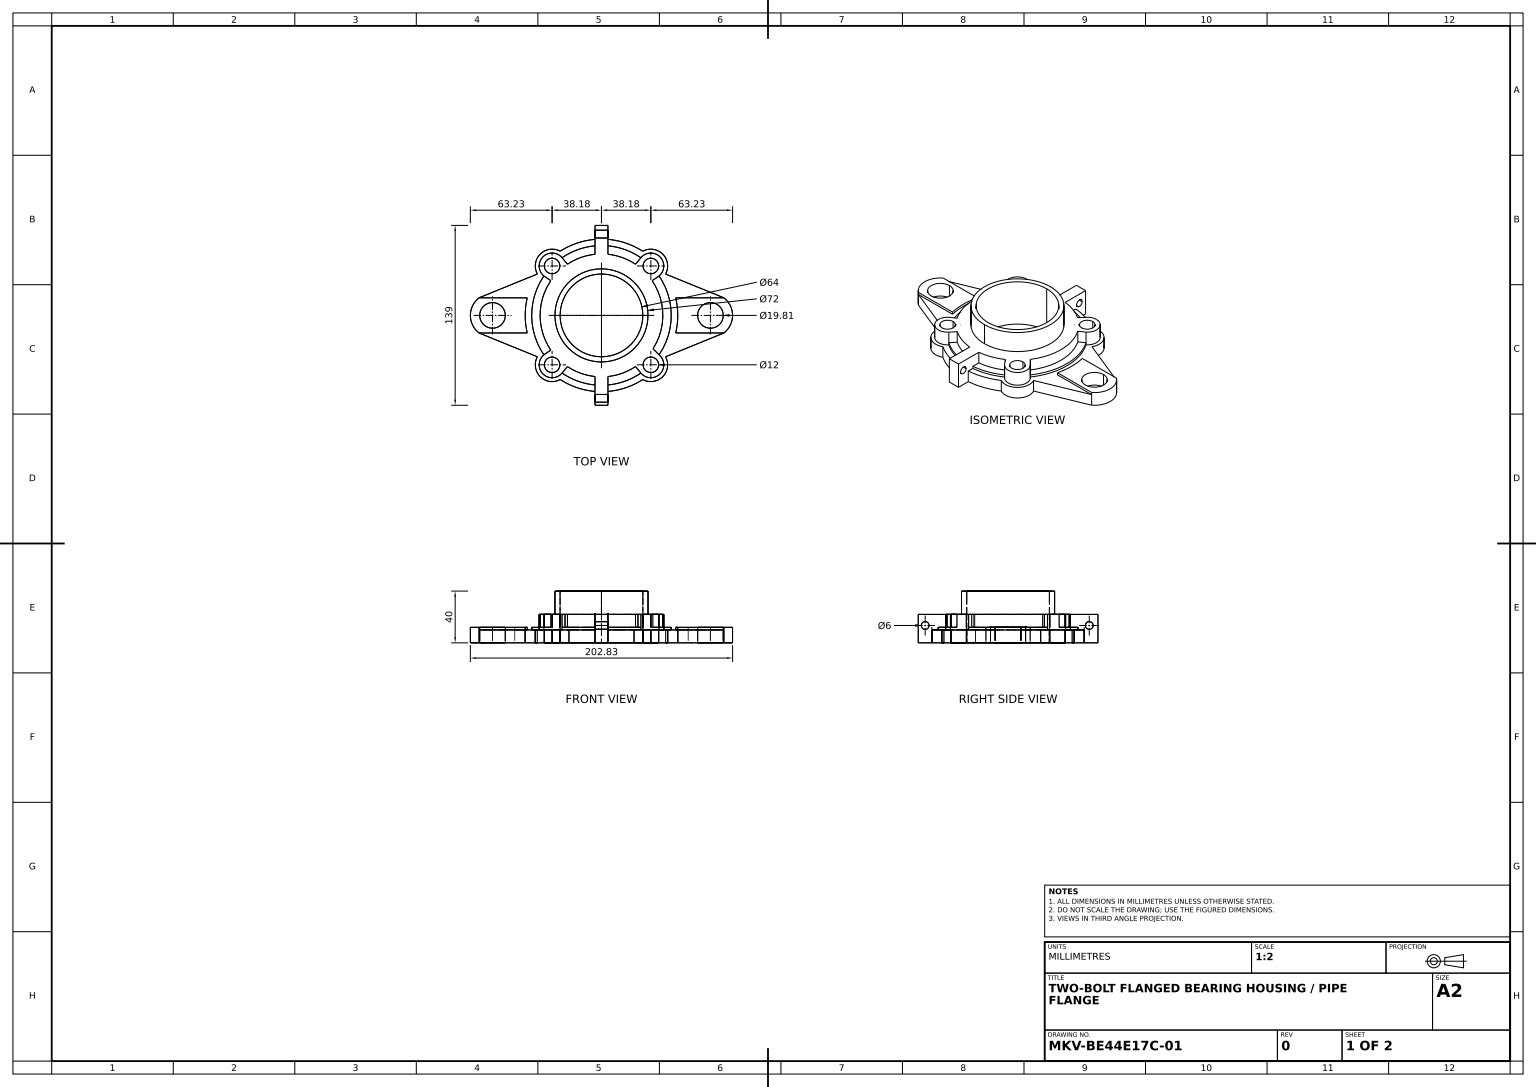
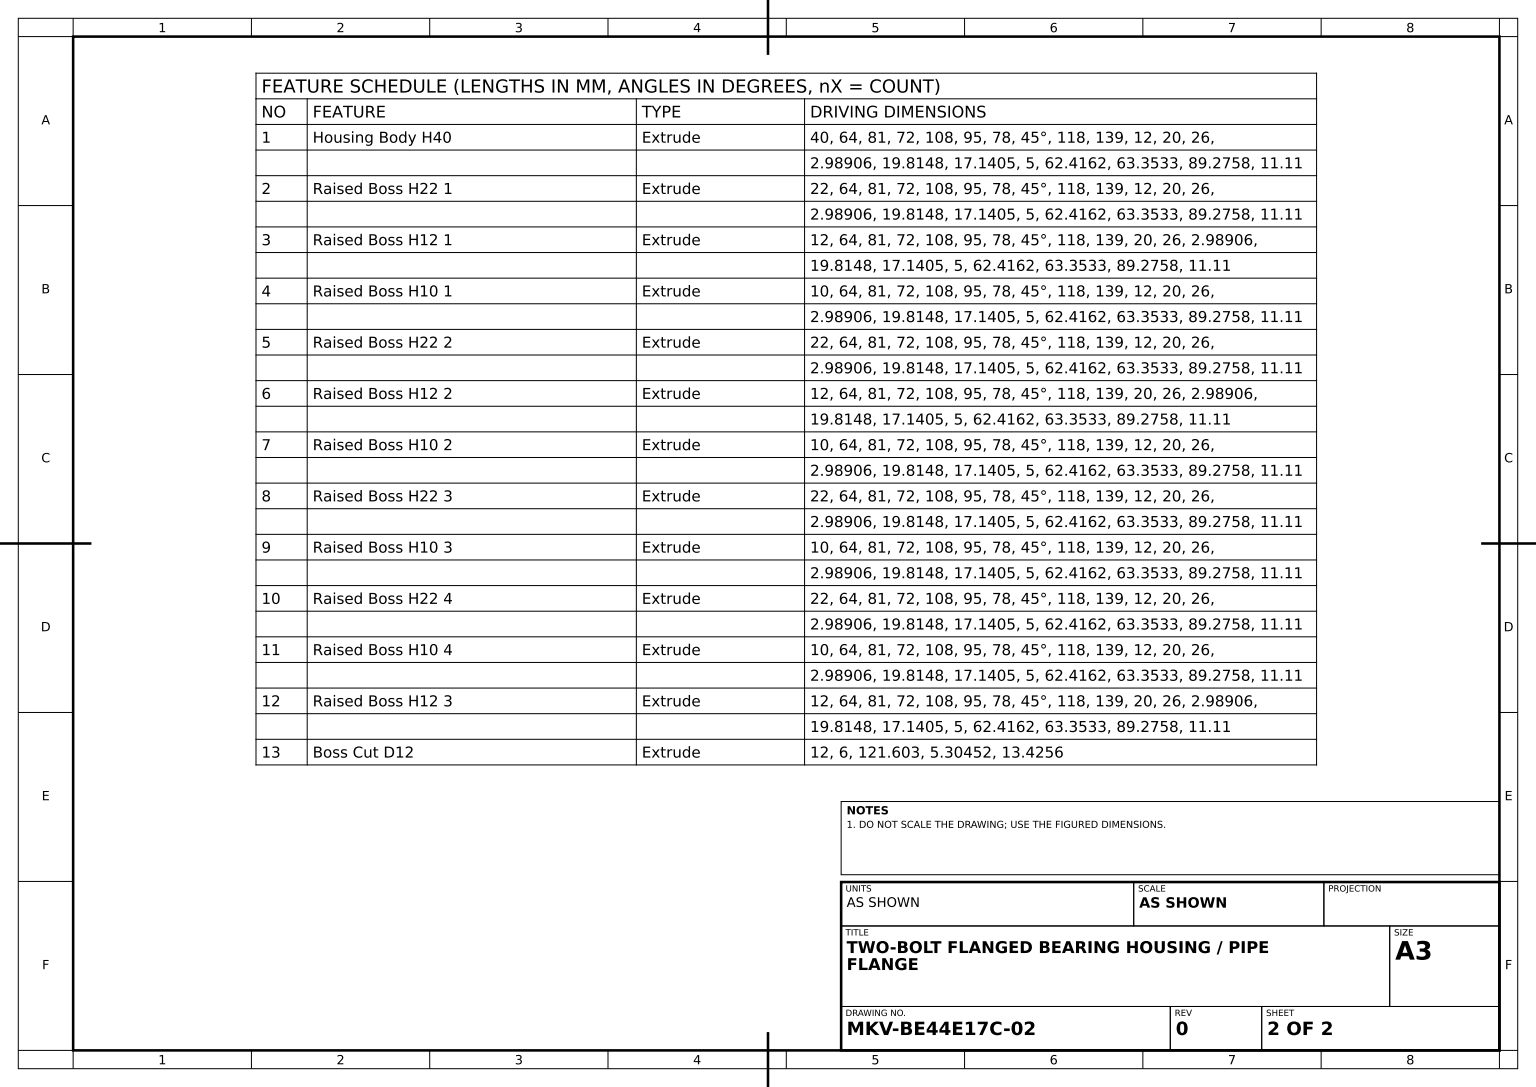
solid
v1 (-49.595662,10,31.95732)
v2 (-49.595662,0,31.95732)
e1 v1 v2 LINE
v3 (-94.736258,10,13.578494)
e2 v1 v3 LINE
v4 (-94.736258,0,13.578494)
e3 v3 v4 LINE
e4 v2 v4 LINE
face PLANE(AX(P(-18.21347,10,44.734463),D(-0.377089462,0,0.926176839),D(0.926176839,0,0.377089462))) [-e1 e2 e3 -e4]
v5 (-39.204854,12,-26.818453)
v6 (-39.204854,12,26.818453)
e5 v5 v6 CIRCLE(AX(P(0,12,0),D(0,1,0),D(0,0,1)),47.5)
v7 (-39.204854,22,26.818453)
e6 v7 v6 LINE
v8 (-39.204854,22,-26.818453)
e7 v8 v7 CIRCLE(AX(P(0,22,0),D(0,1,0),D(0,0,1)),47.5)
e8 v8 v5 LINE
face CYL(AX(P(0,22,0),D(0,-1,0),D(0,0,-1)),47.5) [e5 -e6 -e7 e8]
v9 (5,12,53.76802)
v10 (30.488347,12,44.569729)
e9 v9 v10 CIRCLE(AX(P(0,12,0),D(0,1,0),D(0,0,1)),54)
v11 (26.317093,12,39.543149)
e10 v10 v11 LINE
v12 (5,12,47.236109)
e11 v12 v11 CIRCLE(AX(P(0,12,0),D(0,1,0),D(0,0,1)),47.5)
e12 v12 v9 LINE
face PLANE(AX(P(0,12,0),D(0,1,0),D(0,0,1))) [e9 e10 -e11 e12]
v13 (26.317093,12,-39.543149)
v14 (5,12,-47.236109)
e13 v13 v14 CIRCLE(AX(P(0,12,0),D(0,1,0),D(0,0,1)),47.5)
v15 (30.488347,12,-44.569729)
e14 v15 v13 LINE
v16 (5,12,-53.76802)
e15 v15 v16 CIRCLE(AX(P(0,12,0),D(0,1,0),D(0,0,1)),54)
e16 v14 v16 LINE
face PLANE(AX(P(0,12,0),D(0,1,0),D(0,0,1))) [-e13 -e14 e15 -e16]
v17 (-94.736258,12,13.578494)
v18 (-94.736258,12,-13.578494)
e17 v17 v18 CIRCLE(AX(P(-84.275783,12,0),D(0,-1,0),D(0,0,1)),17.140508)
v19 (-94.736258,10,-13.578494)
e18 v18 v19 LINE
v20 (-94.736258,0,-13.578494)
e19 v19 v20 LINE
e20 v4 v20 CIRCLE(AX(P(-84.275783,0,0),D(0,-1,0),D(0,0,1)),17.140508)
e21 v17 v3 LINE
face CYL(AX(P(-84.275783,12,0),D(0,-1,0),D(0,0,-1)),17.140508) [e17 e18 e19 -e20 -e3 -e21]
v21 (26.317093,22,39.543149)
e22 v21 v11 LINE
v22 (5,22,47.236109)
e23 v22 v21 CIRCLE(AX(P(0,22,0),D(0,1,0),D(0,0,1)),47.5)
e24 v22 v12 LINE
face CYL(AX(P(0,22,0),D(0,-1,0),D(0,0,-1)),47.5) [-e22 -e23 e24 e11]
v23 (39.882032,12,25.80065)
v24 (39.204854,12,-26.818453)
e25 v23 v24 CIRCLE(AX(P(0,12,0),D(0,1,0),D(0,0,1)),47.5)
v25 (39.204854,22,-26.818453)
e26 v25 v24 LINE
v26 (39.882032,22,25.80065)
e27 v26 v25 CIRCLE(AX(P(0,22,0),D(0,1,0),D(0,0,1)),47.5)
e28 v26 v23 LINE
face CYL(AX(P(0,22,0),D(0,-1,0),D(0,0,-1)),47.5) [e25 -e26 -e27 e28]
v27 (-57.416239,12,-13.578494)
v28 (-57.416239,10,-13.578494)
e29 v27 v28 LINE
v29 (-57.416239,12,13.578494)
e30 v27 v29 CIRCLE(AX(P(0,12,0),D(0,1,0),D(0,0,1)),59)
v30 (-57.416239,10,13.578494)
e31 v29 v30 LINE
e32 v28 v30 CIRCLE(AX(P(0,10,0),D(0,1,0),D(0,0,1)),59)
face CYL(AX(P(0,12,0),D(0,-1,0),D(0,0,-1)),59) rev [-e29 e30 e31 -e32]
v31 (84.275783,12,-9.907401)
v32 (84.275783,0,-9.907401)
e33 v31 v32 LINE
v33 (84.275783,0,9.907401)
e34 v33 v32 CIRCLE(AX(P(84.275783,0,0),D(0,1,0),D(0,0,1)),9.907401)
v34 (84.275783,12,9.907401)
e35 v34 v33 LINE
e36 v34 v31 CIRCLE(AX(P(84.275783,12,0),D(0,1,0),D(0,0,1)),9.907401)
face CYL(AX(P(84.275783,12,0),D(0,-1,0),D(0,0,-1)),9.907401) rev [e33 -e34 -e35 e36]
v35 (5,10,53.76802)
e37 v9 v35 LINE
v36 (30.488347,10,44.569729)
e38 v35 v36 CIRCLE(AX(P(0,10,0),D(0,1,0),D(0,0,1)),54)
e39 v10 v36 LINE
face CYL(AX(P(0,12,0),D(0,-1,0),D(0,0,-1)),54) [e37 e38 -e39 -e9]
v37 (-30.488347,22,-44.569729)
v38 (-38.183766,22,-48.183766)
e40 v37 v38 CIRCLE(AX(P(-38.183766,22,-38.183766),D(0,1,0),D(0,0,1)),10)
v39 (-30.488347,12,-44.569729)
e41 v37 v39 LINE
v40 (-30.488347,10,-44.569729)
e42 v39 v40 LINE
v41 (-38.183766,10,-48.183766)
e43 v40 v41 CIRCLE(AX(P(-38.183766,10,-38.183766),D(0,1,0),D(0,0,1)),10)
e44 v38 v41 LINE
face CYL(AX(P(-38.183766,22,-38.183766),D(0,-1,0),D(0,0,-1)),10) [-e40 e41 e42 e43 -e44]
v42 (38.183766,0,44.183766)
v43 (38.183766,0,32.183766)
e45 v42 v43 CIRCLE(AX(P(38.183766,0,38.183766),D(0,1,0),D(0,0,1)),6)
v44 (38.183766,22,44.183766)
e46 v44 v42 LINE
v45 (38.183766,22,32.183766)
e47 v44 v45 CIRCLE(AX(P(38.183766,22,38.183766),D(0,1,0),D(0,0,1)),6)
e48 v45 v43 LINE
face CYL(AX(P(38.183766,22,38.183766),D(0,-1,0),D(0,0,-1)),6) rev [-e45 -e46 e47 e48]
v46 (31.95732,10,-49.595662)
v47 (31.95732,0,-49.595662)
e49 v46 v47 LINE
v48 (5,0,-58.787754)
e50 v47 v48 CIRCLE(AX(P(0,0,0),D(0,1,0),D(0,0,1)),59)
v49 (5,10,-58.787754)
e51 v49 v48 LINE
e52 v46 v49 CIRCLE(AX(P(0,10,0),D(0,1,0),D(0,0,1)),59)
face CYL(AX(P(0,10,0),D(0,-1,0),D(0,0,-1)),59) [e49 e50 -e51 -e52]
v50 (-31.95732,0,49.595662)
e53 v50 v2 CIRCLE(AX(P(-38.183766,0,38.183766),D(0,-1,0),D(0,0,1)),13)
v51 (-31.95732,10,49.595662)
e54 v51 v50 LINE
e55 v51 v1 CIRCLE(AX(P(-38.183766,10,38.183766),D(0,-1,0),D(0,0,1)),13)
face CYL(AX(P(-38.183766,10,38.183766),D(0,-1,0),D(0,0,-1)),13) [-e53 -e54 e55 e1]
v52 (0,40,32)
v53 (0,40,-32)
e56 v52 v53 CIRCLE(AX(P(0,40,0),D(0,1,0),D(0,0,1)),32)
e57 v53 v52 CIRCLE(AX(P(0,40,0),D(0,1,0),D(0,0,1)),32)
v54 (0,40,36)
v55 (0,40,-36)
e58 v54 v55 CIRCLE(AX(P(0,40,0),D(0,1,0),D(0,0,1)),36)
e59 v55 v54 CIRCLE(AX(P(0,40,0),D(0,1,0),D(0,0,1)),36)
face PLANE(AX(P(0,40,0),D(0,1,0),D(0,0,1))) [-e56 -e57] [e58 e59]
v56 (-44.569729,12,-30.488347)
v57 (-44.569729,12,30.488347)
e60 v56 v57 CIRCLE(AX(P(0,12,0),D(0,1,0),D(0,0,1)),54)
e61 v57 v6 LINE
e62 v56 v5 LINE
face PLANE(AX(P(0,12,0),D(0,1,0),D(0,0,1))) [e60 e61 -e5 -e62]
v58 (30.488347,22,44.569729)
e63 v58 v21 LINE
e64 v58 v10 LINE
face PLANE(AX(P(-3.84771,22,3.192981),D(-0.769541956,0,0.638596256),D(0.638596256,0,0.769541956))) [e63 e22 -e10 -e64]
v59 (44.569729,22,30.488347)
e65 v58 v59 CIRCLE(AX(P(38.183766,22,38.183766),D(0,1,0),D(0,0,1)),10)
v60 (44.569729,10,30.488347)
e66 v36 v60 CIRCLE(AX(P(38.183766,10,38.183766),D(0,1,0),D(0,0,1)),10)
v61 (44.569729,12,30.488347)
e67 v61 v60 LINE
e68 v59 v61 LINE
face CYL(AX(P(38.183766,22,38.183766),D(0,-1,0),D(0,0,-1)),10) [-e65 e64 e39 e66 -e67 -e68]
v62 (0,22,-36)
e69 v55 v62 LINE
v63 (0,22,36)
e70 v54 v63 LINE
e71 v63 v62 CIRCLE(AX(P(0,22,0),D(0,1,0),D(0,0,1)),36)
face CYL(AX(P(0,40,0),D(0,-1,0),D(0,0,-1)),36) [-e69 -e58 e70 e71]
v64 (-84.275783,12,9.907401)
v65 (-84.275783,0,9.907401)
e72 v64 v65 LINE
v66 (-84.275783,0,-9.907401)
e73 v65 v66 CIRCLE(AX(P(-84.275783,0,0),D(0,-1,0),D(0,0,1)),9.907401)
v67 (-84.275783,12,-9.907401)
e74 v67 v66 LINE
e75 v64 v67 CIRCLE(AX(P(-84.275783,12,0),D(0,-1,0),D(0,0,1)),9.907401)
face CYL(AX(P(-84.275783,12,0),D(0,-1,0),D(0,0,-1)),9.907401) rev [e72 e73 -e74 -e75]
v68 (0,0,32)
e76 v52 v68 LINE
v69 (0,0,-32)
e77 v69 v68 CIRCLE(AX(P(0,0,0),D(0,1,0),D(0,0,1)),32)
e78 v53 v69 LINE
face CYL(AX(P(0,40,0),D(0,-1,0),D(0,0,-1)),32) rev [e57 e76 -e77 -e78]
e79 v19 v28 LINE
e80 v18 v27 LINE
face PLANE(AX(P(0,12,-13.578494),D(0,0,-1),D(-1,0,0))) [-e79 -e18 e80 e29]
v70 (-38.183766,10,-51.183766)
v71 (-49.595662,10,-31.95732)
e81 v70 v71 CIRCLE(AX(P(-38.183766,10,-38.183766),D(0,1,0),D(0,0,1)),13)
v72 (-38.183766,0,-51.183766)
e82 v70 v72 LINE
v73 (-49.595662,0,-31.95732)
e83 v72 v73 CIRCLE(AX(P(-38.183766,0,-38.183766),D(0,1,0),D(0,0,1)),13)
e84 v71 v73 LINE
face CYL(AX(P(-38.183766,10,-38.183766),D(0,-1,0),D(0,0,-1)),13) [-e81 e82 e83 -e84]
e85 v61 v23 LINE
e86 v59 v26 LINE
face PLANE(AX(P(7.040691,22,-7.040691),D(-0.707106781,0,0.707106781),D(0.707106781,0,0.707106781))) rev [e68 e85 -e28 -e86]
v74 (-38.183766,22,32.183766)
v75 (-38.183766,0,32.183766)
e87 v74 v75 LINE
v76 (-38.183766,22,44.183766)
e88 v76 v74 CIRCLE(AX(P(-38.183766,22,38.183766),D(0,-1,0),D(0,0,1)),6)
v77 (-38.183766,0,44.183766)
e89 v76 v77 LINE
e90 v77 v75 CIRCLE(AX(P(-38.183766,0,38.183766),D(0,-1,0),D(0,0,1)),6)
face CYL(AX(P(-38.183766,22,38.183766),D(0,-1,0),D(0,0,-1)),6) rev [-e87 -e88 e89 e90]
v78 (49.595662,0,31.95732)
v79 (94.736258,0,13.578494)
e91 v78 v79 LINE
v80 (94.736258,10,13.578494)
e92 v80 v79 LINE
v81 (49.595662,10,31.95732)
e93 v81 v80 LINE
e94 v81 v78 LINE
face PLANE(AX(P(18.21347,10,44.734463),D(-0.377089462,0,-0.926176839),D(-0.926176839,0,0.377089462))) rev [e91 -e92 -e93 e94]
v82 (-5,22,-47.236109)
v83 (-5,12,-47.236109)
e95 v82 v83 LINE
v84 (-5,22,-69.536748)
e96 v82 v84 LINE
v85 (-5,0,-69.536748)
e97 v84 v85 LINE
v86 (-5,0,-58.787754)
e98 v86 v85 LINE
v87 (-5,10,-58.787754)
e99 v87 v86 LINE
v88 (-5,10,-53.76802)
e100 v88 v87 LINE
v89 (-5,12,-53.76802)
e101 v89 v88 LINE
e102 v83 v89 LINE
v90 (-5,13.425612,-59.815285)
v91 (-5,13.425612,-65.815285)
e103 v90 v91 CIRCLE(AX(P(-5,13.425612,-62.815285),D(-1,0,0),D(0,0,1)),3)
e104 v91 v90 CIRCLE(AX(P(-5,13.425612,-62.815285),D(-1,0,0),D(0,0,1)),3)
face PLANE(AX(P(-5,22,0),D(-1,0,0),D(0,0,1))) [-e95 e96 e97 -e98 -e99 -e100 -e101 -e102] [-e103 -e104]
v92 (-44.569729,10,-30.488347)
e105 v41 v92 CIRCLE(AX(P(-38.183766,10,-38.183766),D(0,1,0),D(0,0,1)),10)
e106 v56 v92 LINE
v93 (-44.569729,22,-30.488347)
e107 v93 v56 LINE
e108 v38 v93 CIRCLE(AX(P(-38.183766,22,-38.183766),D(0,1,0),D(0,0,1)),10)
face CYL(AX(P(-38.183766,22,-38.183766),D(0,-1,0),D(0,0,-1)),10) [e44 e105 -e106 -e107 -e108]
v94 (-30.488347,22,44.569729)
v95 (-30.488347,12,44.569729)
e109 v94 v95 LINE
v96 (-26.317093,12,39.543149)
e110 v95 v96 LINE
v97 (-26.317093,22,39.543149)
e111 v97 v96 LINE
e112 v94 v97 LINE
face PLANE(AX(P(3.84771,22,3.192981),D(-0.769541956,0,-0.638596256),D(-0.638596256,0,0.769541956))) rev [e109 e110 -e111 -e112]
v98 (94.736258,12,-13.578494)
v99 (94.736258,10,-13.578494)
e113 v98 v99 LINE
v100 (94.736258,12,13.578494)
e114 v100 v98 CIRCLE(AX(P(84.275783,12,0),D(0,1,0),D(0,0,1)),17.140508)
e115 v100 v80 LINE
v101 (94.736258,0,-13.578494)
e116 v79 v101 CIRCLE(AX(P(84.275783,0,0),D(0,1,0),D(0,0,1)),17.140508)
e117 v99 v101 LINE
face CYL(AX(P(84.275783,12,0),D(0,-1,0),D(0,0,-1)),17.140508) [-e113 -e114 e115 e92 e116 -e117]
v102 (57.416239,12,-13.578494)
e118 v98 v102 LINE
v103 (57.416239,12,13.578494)
e119 v103 v102 CIRCLE(AX(P(0,12,0),D(0,1,0),D(0,0,1)),59)
e120 v100 v103 LINE
e121 v31 v34 CIRCLE(AX(P(84.275783,12,0),D(0,1,0),D(0,0,1)),9.907401)
face PLANE(AX(P(0,12,0),D(0,1,0),D(0,0,1))) [e118 -e119 -e120 e114] [-e121 -e36]
v104 (30.488347,10,-44.569729)
v105 (5,10,-53.76802)
e122 v104 v105 CIRCLE(AX(P(0,10,0),D(0,1,0),D(0,0,1)),54)
e123 v16 v105 LINE
e124 v15 v104 LINE
face CYL(AX(P(0,12,0),D(0,-1,0),D(0,0,-1)),54) [e122 -e123 -e15 e124]
e125 v88 v40 CIRCLE(AX(P(0,10,0),D(0,1,0),D(0,0,1)),54)
e126 v89 v39 CIRCLE(AX(P(0,12,0),D(0,1,0),D(0,0,1)),54)
face CYL(AX(P(0,12,0),D(0,-1,0),D(0,0,-1)),54) [e125 -e42 -e126 e101]
v106 (-5,13.425612,61.092276)
v107 (5,13.425612,61.092276)
e127 v106 v107 LINE
v108 (5,13.425612,67.092276)
e128 v107 v108 CIRCLE(AX(P(5,13.425612,64.092276),D(1,0,0),D(0,0,-1)),3)
v109 (-5,13.425612,67.092276)
e129 v109 v108 LINE
e130 v106 v109 CIRCLE(AX(P(-5,13.425612,64.092276),D(1,0,0),D(0,0,-1)),3)
face CYL(AX(P(-7,13.425612,64.092276),D(1,0,0),D(0,0,-1)),3) rev [e127 e128 -e129 -e130]
v110 (5,0,58.787754)
v111 (31.95732,0,49.595662)
e131 v110 v111 CIRCLE(AX(P(0,0,0),D(0,1,0),D(0,0,1)),59)
v112 (31.95732,10,49.595662)
e132 v112 v111 LINE
v113 (5,10,58.787754)
e133 v113 v112 CIRCLE(AX(P(0,10,0),D(0,1,0),D(0,0,1)),59)
e134 v113 v110 LINE
face CYL(AX(P(0,10,0),D(0,-1,0),D(0,0,-1)),59) [e131 -e132 -e133 e134]
v114 (5,13.425612,-65.815285)
v115 (5,13.425612,-59.815285)
e135 v114 v115 CIRCLE(AX(P(5,13.425612,-62.815285),D(1,0,0),D(0,0,-1)),3)
e136 v90 v115 LINE
e137 v91 v114 LINE
face CYL(AX(P(-7,13.425612,-62.815285),D(1,0,0),D(0,0,-1)),3) rev [e135 -e136 e103 e137]
e138 v108 v107 CIRCLE(AX(P(5,13.425612,64.092276),D(1,0,0),D(0,0,-1)),3)
e139 v35 v113 LINE
v116 (5,22,69.463252)
e140 v22 v116 LINE
v117 (5,0,69.463252)
e141 v116 v117 LINE
e142 v110 v117 LINE
face PLANE(AX(P(5,22,0),D(1,0,0),D(0,0,-1))) [-e138 -e128] [-e134 -e139 -e37 -e12 -e24 e140 e141 -e142]
v118 (-26.317093,12,-39.543149)
e143 v39 v118 LINE
e144 v83 v118 CIRCLE(AX(P(0,12,0),D(0,1,0),D(0,0,1)),47.5)
face PLANE(AX(P(0,12,0),D(0,1,0),D(0,0,1))) [e126 e143 -e144 e102]
v119 (-44.569729,22,30.488347)
e145 v119 v57 LINE
e146 v119 v7 LINE
face PLANE(AX(P(0,22,0),D(-0.564599012,0,-0.825365347),D(-0.825365347,0,0.564599012))) [-e61 -e145 e146 e6]
v120 (57.416239,10,-13.578494)
e147 v99 v120 LINE
e148 v102 v120 LINE
face PLANE(AX(P(0,12,-13.578494),D(0,0,1),D(1,0,0))) rev [-e118 e113 e147 -e148]
e149 v62 v63 CIRCLE(AX(P(0,22,0),D(0,1,0),D(0,0,1)),36)
face CYL(AX(P(0,40,0),D(0,-1,0),D(0,0,-1)),36) [-e59 e69 e149 -e70]
v121 (57.416239,10,13.578494)
e150 v121 v120 CIRCLE(AX(P(0,10,0),D(0,1,0),D(0,0,1)),59)
e151 v103 v121 LINE
face CYL(AX(P(0,12,0),D(0,-1,0),D(0,0,-1)),59) rev [e119 e148 -e150 -e151]
v122 (38.183766,10,-51.183766)
v123 (38.183766,0,-51.183766)
e152 v122 v123 LINE
e153 v47 v123 CIRCLE(AX(P(38.183766,0,-38.183766),D(0,-1,0),D(0,0,1)),13)
e154 v46 v122 CIRCLE(AX(P(38.183766,10,-38.183766),D(0,-1,0),D(0,0,1)),13)
face CYL(AX(P(38.183766,10,-38.183766),D(0,-1,0),D(0,0,-1)),13) [e152 -e153 -e49 e154]
v124 (26.317093,22,-39.543149)
e155 v124 v13 LINE
v125 (30.488347,22,-44.569729)
e156 v125 v124 LINE
e157 v125 v15 LINE
face PLANE(AX(P(-3.84771,22,-3.192981),D(0.769541956,0,0.638596256),D(0.638596256,0,-0.769541956))) rev [e14 -e155 -e156 e157]
v126 (5,22,-69.536748)
e158 v84 v126 LINE
v127 (5,0,-69.536748)
e159 v126 v127 LINE
e160 v85 v127 LINE
face PLANE(AX(P(0,22,-69.536748),D(0,0,-1),D(-1,0,0))) [e158 e159 -e160 -e97]
v128 (38.183766,22,-32.183766)
v129 (38.183766,0,-32.183766)
e161 v128 v129 LINE
v130 (38.183766,0,-44.183766)
e162 v129 v130 CIRCLE(AX(P(38.183766,0,-38.183766),D(0,-1,0),D(0,0,1)),6)
v131 (38.183766,22,-44.183766)
e163 v131 v130 LINE
e164 v128 v131 CIRCLE(AX(P(38.183766,22,-38.183766),D(0,-1,0),D(0,0,1)),6)
face CYL(AX(P(38.183766,22,-38.183766),D(0,-1,0),D(0,0,-1)),6) rev [e161 e162 -e163 -e164]
v132 (38.183766,10,-48.183766)
v133 (44.569729,10,-30.488347)
e165 v132 v133 CIRCLE(AX(P(38.183766,10,-38.183766),D(0,-1,0),D(0,0,1)),10)
v134 (38.183766,22,-48.183766)
e166 v134 v132 LINE
v135 (44.569729,22,-30.488347)
e167 v134 v135 CIRCLE(AX(P(38.183766,22,-38.183766),D(0,-1,0),D(0,0,1)),10)
v136 (44.569729,12,-30.488347)
e168 v135 v136 LINE
e169 v136 v133 LINE
face CYL(AX(P(38.183766,22,-38.183766),D(0,-1,0),D(0,0,-1)),10) [-e165 -e166 e167 e168 e169]
v137 (-5,12,53.76802)
v138 (-5,10,53.76802)
e170 v137 v138 LINE
e171 v95 v137 CIRCLE(AX(P(0,12,0),D(0,1,0),D(0,0,1)),54)
v139 (-30.488347,10,44.569729)
e172 v95 v139 LINE
e173 v139 v138 CIRCLE(AX(P(0,10,0),D(0,1,0),D(0,0,1)),54)
face CYL(AX(P(0,12,0),D(0,-1,0),D(0,0,-1)),54) [-e170 -e171 e172 e173]
v140 (-31.95732,0,-49.595662)
e174 v86 v140 CIRCLE(AX(P(0,0,0),D(0,1,0),D(0,0,1)),59)
v141 (-31.95732,10,-49.595662)
e175 v141 v140 LINE
e176 v87 v141 CIRCLE(AX(P(0,10,0),D(0,1,0),D(0,0,1)),59)
face CYL(AX(P(0,10,0),D(0,-1,0),D(0,0,-1)),59) [e174 -e175 -e176 e99]
e177 v111 v78 CIRCLE(AX(P(38.183766,0,38.183766),D(0,1,0),D(0,0,1)),13)
e178 v112 v81 CIRCLE(AX(P(38.183766,10,38.183766),D(0,1,0),D(0,0,1)),13)
face CYL(AX(P(38.183766,10,38.183766),D(0,-1,0),D(0,0,-1)),13) [e132 e177 -e94 -e178]
v142 (-38.183766,22,-32.183766)
v143 (-38.183766,22,-44.183766)
e179 v142 v143 CIRCLE(AX(P(-38.183766,22,-38.183766),D(0,1,0),D(0,0,1)),6)
e180 v143 v142 CIRCLE(AX(P(-38.183766,22,-38.183766),D(0,1,0),D(0,0,1)),6)
e181 v45 v44 CIRCLE(AX(P(38.183766,22,38.183766),D(0,1,0),D(0,0,1)),6)
e182 v74 v76 CIRCLE(AX(P(-38.183766,22,38.183766),D(0,-1,0),D(0,0,1)),6)
v144 (-26.317093,22,-39.543149)
e183 v37 v144 LINE
e184 v93 v8 LINE
e185 v94 v119 CIRCLE(AX(P(-38.183766,22,38.183766),D(0,-1,0),D(0,0,1)),10)
v145 (-5,22,47.236109)
e186 v97 v145 CIRCLE(AX(P(0,22,0),D(0,1,0),D(0,0,1)),47.5)
v146 (-5,22,69.463252)
e187 v145 v146 LINE
e188 v146 v116 LINE
e189 v135 v25 LINE
e190 v125 v134 CIRCLE(AX(P(38.183766,22,-38.183766),D(0,-1,0),D(0,0,1)),10)
v147 (5,22,-47.236109)
e191 v124 v147 CIRCLE(AX(P(0,22,0),D(0,1,0),D(0,0,1)),47.5)
e192 v147 v126 LINE
e193 v82 v144 CIRCLE(AX(P(0,22,0),D(0,1,0),D(0,0,1)),47.5)
e194 v131 v128 CIRCLE(AX(P(38.183766,22,-38.183766),D(0,-1,0),D(0,0,1)),6)
face PLANE(AX(P(0,22,0),D(0,1,0),D(0,0,1))) [-e179 -e180] [-e181 -e47] [e182 e88] [-e183 e40 e108 e184 e7 -e146 -e185 e112 e186 e187 e188 -e140 e23 -e63 e65 e86 e27 -e189 -e167 -e190 e156 e191 e192 -e158 -e96 e193] [e164 e194] [-e71 -e149]
e195 v115 v114 CIRCLE(AX(P(5,13.425612,-62.815285),D(1,0,0),D(0,0,-1)),3)
e196 v105 v49 LINE
e197 v48 v127 LINE
e198 v147 v14 LINE
face PLANE(AX(P(5,22,0),D(-1,0,0),D(0,0,1))) rev [-e195 -e135] [e123 e196 e51 e197 -e159 -e192 e198 e16]
v148 (-5,0,69.463252)
e199 v146 v148 LINE
e200 v148 v117 LINE
face PLANE(AX(P(0,22,69.463252),D(0,0,-1),D(-1,0,0))) rev [-e188 e199 e200 -e141]
e201 v61 v136 CIRCLE(AX(P(0,12,0),D(0,1,0),D(0,0,1)),54)
e202 v136 v24 LINE
face PLANE(AX(P(0,12,0),D(0,1,0),D(0,0,1))) [-e85 e201 e202 -e25]
e203 v32 v33 CIRCLE(AX(P(84.275783,0,0),D(0,1,0),D(0,0,1)),9.907401)
face CYL(AX(P(84.275783,12,0),D(0,-1,0),D(0,0,-1)),9.907401) rev [e35 -e203 -e33 e121]
face PLANE(AX(P(0,22,0),D(0.564599012,0,0.825365347),D(0.825365347,0,-0.564599012))) [e189 e26 -e202 -e168]
e204 v144 v118 LINE
face CYL(AX(P(0,22,0),D(0,-1,0),D(0,0,-1)),47.5) [e95 e144 -e204 -e193]
e205 v68 v69 CIRCLE(AX(P(0,0,0),D(0,1,0),D(0,0,1)),32)
face CYL(AX(P(0,40,0),D(0,-1,0),D(0,0,-1)),32) rev [e78 -e205 -e76 e56]
face PLANE(AX(P(0,22,0),D(0.564599012,0,-0.825365347),D(-0.825365347,0,-0.564599012))) rev [e62 -e8 -e184 e107]
e206 v109 v106 CIRCLE(AX(P(-5,13.425612,64.092276),D(1,0,0),D(0,0,-1)),3)
face CYL(AX(P(-7,13.425612,64.092276),D(1,0,0),D(0,0,-1)),3) rev [e138 -e127 -e206 e129]
v149 (-5,10,58.787754)
v150 (-5,0,58.787754)
e207 v149 v150 LINE
e208 v51 v149 CIRCLE(AX(P(0,10,0),D(0,1,0),D(0,0,1)),59)
e209 v50 v150 CIRCLE(AX(P(0,0,0),D(0,1,0),D(0,0,1)),59)
face CYL(AX(P(0,10,0),D(0,-1,0),D(0,0,-1)),59) [-e207 -e208 e54 e209]
v151 (-5,12,47.236109)
e210 v151 v137 LINE
e211 v96 v151 CIRCLE(AX(P(0,12,0),D(0,1,0),D(0,0,1)),47.5)
face PLANE(AX(P(0,12,0),D(0,1,0),D(0,0,1))) [-e110 e171 -e210 -e211]
e212 v104 v132 CIRCLE(AX(P(38.183766,10,-38.183766),D(0,-1,0),D(0,0,1)),10)
e213 v60 v133 CIRCLE(AX(P(0,10,0),D(0,1,0),D(0,0,1)),54)
e214 v80 v121 LINE
v152 (49.595662,10,-31.95732)
e215 v152 v99 LINE
e216 v122 v152 CIRCLE(AX(P(38.183766,10,-38.183766),D(0,-1,0),D(0,0,1)),13)
face PLANE(AX(P(0,10,0),D(0,1,0),D(0,0,1))) [-e196 -e122 e212 e165 -e213 -e66 -e38 e139 e133 e178 e93 e214 e150 -e147 -e215 -e216 -e154 e52]
e217 v130 v129 CIRCLE(AX(P(38.183766,0,-38.183766),D(0,-1,0),D(0,0,1)),6)
face CYL(AX(P(38.183766,22,-38.183766),D(0,-1,0),D(0,0,-1)),6) rev [e217 -e161 -e194 e163]
v153 (-44.569729,10,30.488347)
e218 v57 v153 LINE
e219 v139 v153 CIRCLE(AX(P(-38.183766,10,38.183766),D(0,-1,0),D(0,0,1)),10)
face CYL(AX(P(-38.183766,22,38.183766),D(0,-1,0),D(0,0,-1)),10) [e145 e218 -e219 -e172 -e109 e185]
face CYL(AX(P(0,12,0),D(0,-1,0),D(0,0,-1)),54) [e67 e213 -e169 -e201]
face PLANE(AX(P(0,12,13.578494),D(0,0,1),D(1,0,0))) [e151 -e214 -e115 e120]
e220 v75 v77 CIRCLE(AX(P(-38.183766,0,38.183766),D(0,-1,0),D(0,0,1)),6)
e221 v43 v42 CIRCLE(AX(P(38.183766,0,38.183766),D(0,1,0),D(0,0,1)),6)
v154 (-38.183766,0,-44.183766)
v155 (-38.183766,0,-32.183766)
e222 v154 v155 CIRCLE(AX(P(-38.183766,0,-38.183766),D(0,1,0),D(0,0,1)),6)
e223 v155 v154 CIRCLE(AX(P(-38.183766,0,-38.183766),D(0,1,0),D(0,0,1)),6)
e224 v66 v65 CIRCLE(AX(P(-84.275783,0,0),D(0,-1,0),D(0,0,1)),9.907401)
e225 v150 v148 LINE
e226 v73 v20 LINE
e227 v140 v72 CIRCLE(AX(P(-38.183766,0,-38.183766),D(0,1,0),D(0,0,1)),13)
v156 (49.595662,0,-31.95732)
e228 v123 v156 CIRCLE(AX(P(38.183766,0,-38.183766),D(0,-1,0),D(0,0,1)),13)
e229 v156 v101 LINE
face PLANE(AX(P(0,0,0),D(0,1,0),D(0,0,1))) rev [-e90 -e220] [e45 e221] [e34 e203] [e222 e223] [-e73 -e224] [e205 e77] [-e131 e142 -e200 -e225 -e209 e53 e4 e20 -e226 -e83 -e227 -e174 e98 e160 -e197 -e50 e153 e228 e229 -e116 -e91 -e177] [-e162 -e217]
e230 v152 v156 LINE
face PLANE(AX(P(18.21347,10,-44.734463),D(0.377089462,0,-0.926176839),D(-0.926176839,0,-0.377089462))) [e215 e117 -e229 -e230]
e231 v92 v153 CIRCLE(AX(P(0,10,0),D(0,1,0),D(0,0,1)),54)
face CYL(AX(P(0,12,0),D(0,-1,0),D(0,0,-1)),54) [-e60 e106 e231 -e218]
e232 v17 v29 LINE
e233 v67 v64 CIRCLE(AX(P(-84.275783,12,0),D(0,-1,0),D(0,0,1)),9.907401)
face PLANE(AX(P(0,12,0),D(0,1,0),D(0,0,1))) [-e80 -e17 e232 -e30] [e233 e75]
e234 v145 v151 LINE
face CYL(AX(P(0,22,0),D(0,-1,0),D(0,0,-1)),47.5) [e211 -e234 -e186 e111]
face PLANE(AX(P(3.84771,22,-3.192981),D(0.769541956,0,-0.638596256),D(-0.638596256,0,-0.769541956))) [-e143 -e41 e183 e204]
face CYL(AX(P(-7,13.425612,-62.815285),D(1,0,0),D(0,0,-1)),3) rev [e136 e195 -e137 e104]
face CYL(AX(P(0,22,0),D(0,-1,0),D(0,0,-1)),47.5) [-e191 e155 e13 -e198]
face CYL(AX(P(38.183766,10,-38.183766),D(0,-1,0),D(0,0,-1)),13) [e216 e230 -e228 -e152]
face CYL(AX(P(-38.183766,22,38.183766),D(0,-1,0),D(0,0,-1)),6) rev [e87 e220 -e89 -e182]
face CYL(AX(P(-84.275783,12,0),D(0,-1,0),D(0,0,-1)),9.907401) rev [e74 e224 -e72 -e233]
e235 v141 v70 CIRCLE(AX(P(-38.183766,10,-38.183766),D(0,1,0),D(0,0,1)),13)
e236 v71 v19 LINE
e237 v3 v30 LINE
e238 v138 v149 LINE
face PLANE(AX(P(0,10,0),D(0,1,0),D(0,0,1))) [-e105 -e43 -e125 e100 e176 e235 e81 e236 e79 e32 -e237 -e2 -e55 e208 -e238 -e173 e219 -e231]
e239 v143 v154 LINE
e240 v142 v155 LINE
face CYL(AX(P(-38.183766,22,-38.183766),D(0,-1,0),D(0,0,-1)),6) rev [e179 e239 -e223 -e240]
face CYL(AX(P(38.183766,22,-38.183766),D(0,-1,0),D(0,0,-1)),10) [e166 -e212 -e124 -e157 e190]
face PLANE(AX(P(0,12,13.578494),D(0,0,-1),D(-1,0,0))) rev [-e232 e21 e237 -e31]
face CYL(AX(P(-38.183766,22,-38.183766),D(0,-1,0),D(0,0,-1)),6) rev [e180 e240 -e222 -e239]
face PLANE(AX(P(-18.21347,10,-44.734463),D(0.377089462,0,0.926176839),D(0.926176839,0,-0.377089462))) rev [-e19 -e236 e84 e226]
face CYL(AX(P(-38.183766,10,-38.183766),D(0,-1,0),D(0,0,-1)),13) [-e235 e175 e227 -e82]
face PLANE(AX(P(-5,22,0),D(1,0,0),D(0,0,-1))) rev [e225 -e199 -e187 e234 e210 e170 e238 e207] [e206 e130]
face CYL(AX(P(38.183766,22,38.183766),D(0,-1,0),D(0,0,-1)),6) rev [-e221 -e48 e181 e46]
